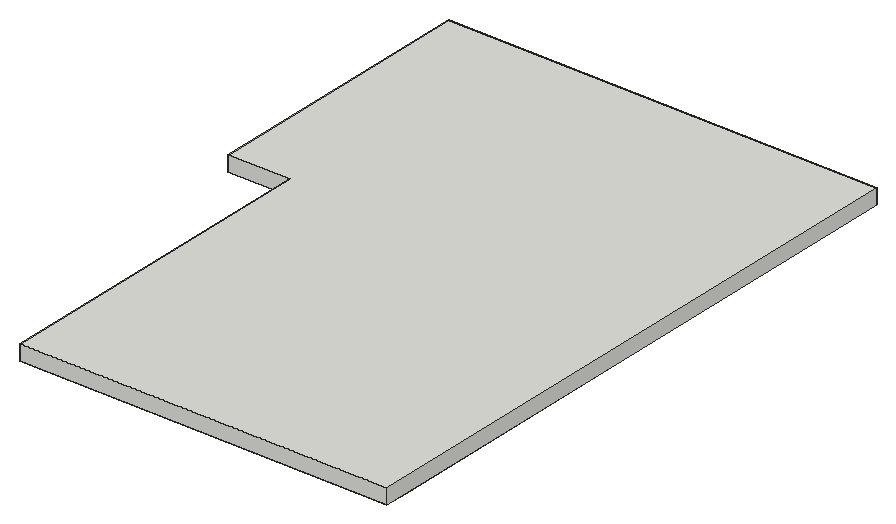
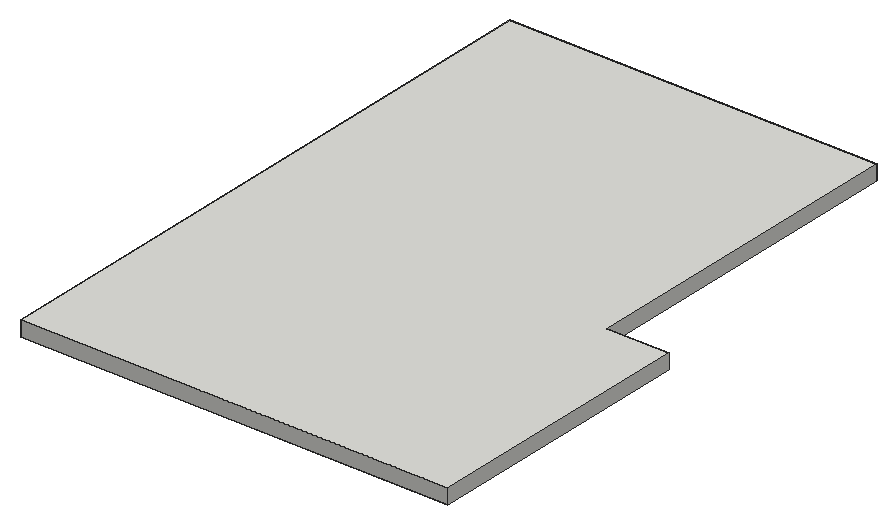
# SketchUp Ruby script. Lengths in inches.
U = 1.inch
M = Sketchup.active_model
def pt(a) = Geom::Point3d.new(a.map { |v| v * U })
def face(e, loops, mat)
  f = e.add_face(loops[0].map { |a| pt(a) })
  loops[1..].each { |l| e.add_face(l.map { |a| pt(a) }).erase! }
  f.material = f.back_material = mat if mat
  f
end
# faces: each face lists its corners as indices into pts; further lists are holes
def faces(e, pts, list, mat = nil) = list.each { |f| face(e, (f[0].is_a?(Array) ? f : [f]).map { |l| l.map { |i| pts[i] } }, mat) }
# xy, xz, yz: faces in a plane at the given z, y or x. An outline is a flat list of corners, or four numbers for a rectangle; further outlines are holes
def ring(l) = l.size == 4 ? [[l[0], l[1]], [l[2], l[1]], [l[2], l[3]], [l[0], l[3]]] : l.each_slice(2).to_a
def flat(e, list, mat, &to3) = list.each { |f| face(e, (f[0].is_a?(Array) ? f : [f]).map { |l| ring(l).map { |u, v| to3.(u, v) } }, mat) }
def xy(e, z, list, mat = nil) = flat(e, list, mat) { |x, y| [x, y, z] }
def xz(e, y, list, mat = nil) = flat(e, list, mat) { |x, z| [x, y, z] }
def yz(e, x, list, mat = nil) = flat(e, list, mat) { |y, z| [x, y, z] }
def lines(e, pts, list) = list.each { |a, b| e.add_line(pt(pts[a]), pt(pts[b])) }
# prism: a flat outline (further loops are holes) pulled along v
def prism(e, loops, v, mat = nil)
  f = face(e, loops, mat); d = Geom::Vector3d.new(v.map { |x| x * U })
  f.pushpull(f.normal.samedirection?(d) ? d.length : -d.length)
end
def box(e, o, s, mat = nil) = prism(e, [[o, [o[0] + s[0], o[1], o[2]], [o[0] + s[0], o[1] + s[1], o[2]], [o[0], o[1] + s[1], o[2]]]], [0, 0, s[2]], mat)
def at(x, y, z, deg = 0) = Geom::Transformation.translation(pt([x, y, z])) * Geom::Transformation.rotation(ORIGIN, Z_AXIS, deg.degrees)
def axes(o, x, y, z) = Geom::Transformation.new([*x, 0, *y, 0, *z, 0, *pt(o).to_a, 1])
def part(name) = M.definitions.add(name)
# library, detail: a bought-in or finely detailed component or shape, given as its bounding box
def library(name, o, s) = part(name).tap { |d| box(d.entities, o, s) }
def detail(e, o, s) = box(e.add_group.entities, o, s)
def put(e, d, t, mat = nil) = e.add_instance(d, t).tap { |i| i.material = mat if mat }
def group(e, t, mat = nil) = e.add_group.tap { |g| g.transformation = t; g.material = mat if mat }.entities
root = M.entities
M.materials.add("False ceiling Light").color = [250, 225, 158]
M.materials.add("[Wood Veneer 01]3").color = [120, 70, 37]
c1 = library("Group\#28",[0,0,0],[152,89,0.5])
c2 = library("Group\#27",[0,0,0],[125,62,0.75])
xy(root,121,[[[75.29,35.75,144.17,35.75,144.21,35.76,144.3,35.76,144.34,35.77,144.38,35.77,144.42,35.78,144.47,35.78,144.55,35.8,144.59,35.8,144.63,35.8125,144.68,35.82,144.92,35.88,144.96,35.9,145.04,35.92,145.08,35.9375,145.125,35.95,145.16,35.97,145.2,35.98,145.24,36,145.28,36.01,145.4,36.07,145.4375,36.09,145.48,36.1,145.51,36.125,145.55,36.14,145.59,36.16,145.625,36.1875,145.66,36.21,145.7,36.23,145.73,36.25,145.77,36.27,145.81,36.3,145.84,36.32,145.875,36.35,145.91,36.37,145.94,36.4,145.98,36.42,146.01,36.45,146.05,36.47,146.14,36.56,146.17,36.58,146.21,36.61,146.39,36.79,146.42,36.83,146.44,36.86,146.53,36.95,146.55,36.99,146.58,37.02,146.6,37.06,146.63,37.09,146.65,37.125,146.68,37.16,146.7,37.19,146.73,37.23,146.75,37.27,146.77,37.3,146.79,37.34,146.8125,37.375,146.84,37.41,146.86,37.45,146.875,37.49,146.9,37.52,146.91,37.5625,146.93,37.6,146.99,37.72,147,37.76,147.02,37.8,147.03,37.84,147.05,37.875,147.0625,37.92,147.08,37.96,147.1,38.04,147.12,38.08,147.18,38.32,147.1875,38.37,147.2,38.41,147.2,38.45,147.22,38.53,147.22,38.58,147.23,38.62,147.23,38.66,147.24,38.7,147.24,38.79,147.25,38.83,147.25,171.17,147.24,171.21,147.24,171.3,147.23,171.34,147.23,171.38,147.22,171.42,147.22,171.47,147.2,171.55,147.2,171.59,147.1875,171.63,147.18,171.68,147.12,171.92,147.1,171.96,147.08,172.04,147.0625,172.08,147.05,172.125,147.03,172.16,147.02,172.2,147,172.24,146.99,172.28,146.93,172.4,146.91,172.4375,146.9,172.48,146.875,172.51,146.86,172.55,146.84,172.59,146.8125,172.625,146.79,172.66,146.77,172.7,146.75,172.73,146.73,172.77,146.7,172.81,146.68,172.84,146.65,172.875,146.63,172.91,146.6,172.94,146.58,172.98,146.55,173.01,146.53,173.05,146.44,173.14,146.42,173.17,146.39,173.21,146.21,173.39,146.17,173.42,146.14,173.44,146.05,173.53,146.01,173.55,145.98,173.58,145.94,173.6,145.91,173.63,145.875,173.65,145.84,173.68,145.81,173.7,145.77,173.73,145.73,173.75,145.7,173.77,145.66,173.79,145.625,173.8125,145.59,173.84,145.55,173.86,145.51,173.875,145.48,173.9,145.4375,173.91,145.4,173.93,145.28,173.99,145.24,174,145.2,174.02,145.16,174.03,145.125,174.05,145.08,174.0625,145.04,174.08,144.96,174.1,144.92,174.12,144.68,174.18,144.63,174.1875,144.59,174.2,144.55,174.2,144.47,174.22,144.42,174.22,144.38,174.23,144.34,174.23,144.3,174.24,144.21,174.24,144.17,174.25,75.29,174.25,74.58,174.2,74.16,174.12,73.76,173.99,73.38,173.8,73.03,173.5625,72.72,173.28,72.4375,172.97,72.2,172.62,72.01,172.24,71.88,171.84,71.8,171.42,71.75,170.71,71.75,39.29,71.8,38.58,71.88,38.16,72.01,37.76,72.2,37.38,72.4375,37.03,72.72,36.72,73.03,36.4375,73.38,36.2,73.76,36.01,74.16,35.88,74.58,35.8],[92.62,42.5,91.86,42.54,91.67,42.5625,91.48,42.58,91.3,42.6,90.92,42.65,90.54,42.71,90.36,42.74,90.17,42.78,89.99,42.82,89.8,42.86,89.62,42.9,89.43,42.95,89.25,42.99,89.0625,43.04,88.88,43.1,88.7,43.15,88.16,43.33,87.98,43.4,87.8,43.46,87.45,43.6,87.28,43.68,87.1,43.75,86.76,43.91,86.59,44,86.42,44.08,85.91,44.35,85.75,44.44,85.59,44.54,85.42,44.64,84.94,44.94,84.79,45.05,84.63,45.16,84.48,45.27,84.32,45.38,84.17,45.5,84.02,45.61,83.73,45.85,83.58,45.97,83.4375,46.1,83.3,46.22,82.88,46.61,82.75,46.75,82.61,46.88,82.22,47.3,82.1,47.4375,81.97,47.58,81.85,47.73,81.61,48.02,81.5,48.17,81.38,48.32,81.27,48.48,81.16,48.63,81.05,48.79,80.94,48.94,80.64,49.42,80.54,49.59,80.44,49.75,80.35,49.91,80.08,50.42,80,50.59,79.91,50.76,79.75,51.1,79.68,51.28,79.6,51.45,79.46,51.8,79.4,51.98,79.33,52.16,79.15,52.7,79.1,52.88,79.04,53.0625,78.99,53.25,78.95,53.43,78.9,53.62,78.86,53.8,78.82,53.99,78.78,54.17,78.74,54.36,78.71,54.54,78.65,54.92,78.6,55.3,78.58,55.48,78.5625,55.67,78.54,55.86,78.5,56.62,78.5,153.38,78.54,154.14,78.5625,154.33,78.58,154.52,78.6,154.7,78.65,155.08,78.71,155.46,78.74,155.64,78.78,155.83,78.82,156.01,78.86,156.2,78.9,156.38,78.95,156.57,78.99,156.75,79.04,156.9375,79.1,157.12,79.15,157.3,79.33,157.84,79.4,158.02,79.46,158.2,79.6,158.55,79.68,158.72,79.75,158.9,79.91,159.24,80,159.41,80.08,159.58,80.35,160.09,80.44,160.25,80.54,160.41,80.64,160.58,80.94,161.06,81.05,161.21,81.16,161.37,81.27,161.52,81.38,161.68,81.5,161.83,81.61,161.98,81.85,162.27,81.97,162.42,82.1,162.5625,82.22,162.7,82.61,163.12,82.75,163.25,82.88,163.39,83.3,163.78,83.4375,163.9,83.58,164.03,83.73,164.15,84.02,164.39,84.17,164.5,84.32,164.62,84.48,164.73,84.63,164.84,84.79,164.95,84.94,165.06,85.42,165.36,85.59,165.46,85.75,165.56,85.91,165.65,86.42,165.92,86.59,166,86.76,166.09,87.1,166.25,87.28,166.32,87.45,166.4,87.8,166.54,87.98,166.6,88.16,166.67,88.7,166.85,88.88,166.9,89.0625,166.96,89.25,167.01,89.43,167.05,89.62,167.1,89.8,167.14,89.99,167.18,90.17,167.22,90.36,167.26,90.54,167.29,90.92,167.35,91.3,167.4,91.48,167.42,91.67,167.4375,91.86,167.46,92.62,167.5,126.38,167.5,127.14,167.46,127.33,167.4375,127.52,167.42,127.7,167.4,128.08,167.35,128.46,167.29,128.64,167.26,128.83,167.22,129.01,167.18,129.2,167.14,129.38,167.1,129.57,167.05,129.75,167.01,129.9375,166.96,130.12,166.9,130.3,166.85,130.84,166.67,131.02,166.6,131.2,166.54,131.55,166.4,131.72,166.32,131.9,166.25,132.24,166.09,132.41,166,132.58,165.92,133.09,165.65,133.25,165.56,133.41,165.46,133.58,165.36,134.06,165.06,134.21,164.95,134.37,164.84,134.52,164.73,134.68,164.62,134.83,164.5,134.98,164.39,135.27,164.15,135.42,164.03,135.5625,163.9,135.7,163.78,136.12,163.39,136.25,163.25,136.39,163.12,136.78,162.7,136.9,162.5625,137.03,162.42,137.15,162.27,137.39,161.98,137.5,161.83,137.62,161.68,137.73,161.52,137.84,161.37,137.95,161.21,138.06,161.06,138.36,160.58,138.46,160.41,138.56,160.25,138.65,160.09,138.92,159.58,139,159.41,139.09,159.24,139.25,158.9,139.32,158.72,139.4,158.55,139.54,158.2,139.6,158.02,139.67,157.84,139.85,157.3,139.9,157.12,139.96,156.9375,140.01,156.75,140.05,156.57,140.1,156.38,140.14,156.2,140.18,156.01,140.22,155.83,140.26,155.64,140.29,155.46,140.35,155.08,140.4,154.7,140.42,154.52,140.4375,154.33,140.46,154.14,140.5,153.38,140.5,56.62,140.46,55.86,140.4375,55.67,140.42,55.48,140.4,55.3,140.35,54.92,140.29,54.54,140.26,54.36,140.22,54.17,140.18,53.99,140.14,53.8,140.1,53.62,140.05,53.43,140.01,53.25,139.96,53.0625,139.9,52.88,139.85,52.7,139.67,52.16,139.6,51.98,139.54,51.8,139.4,51.45,139.32,51.28,139.25,51.1,139.09,50.76,139,50.59,138.92,50.42,138.65,49.91,138.56,49.75,138.46,49.59,138.36,49.42,138.06,48.94,137.95,48.79,137.84,48.63,137.73,48.48,137.62,48.32,137.5,48.17,137.39,48.02,137.15,47.73,137.03,47.58,136.9,47.4375,136.78,47.3,136.39,46.88,136.25,46.75,136.12,46.61,135.7,46.22,135.5625,46.1,135.42,45.97,135.27,45.85,134.98,45.61,134.83,45.5,134.68,45.38,134.52,45.27,134.37,45.16,134.21,45.05,134.06,44.94,133.58,44.64,133.41,44.54,133.25,44.44,133.09,44.35,132.58,44.08,132.41,44,132.24,43.91,131.9,43.75,131.72,43.68,131.55,43.6,131.2,43.46,131.02,43.4,130.84,43.33,130.3,43.15,130.12,43.1,129.9375,43.04,129.75,42.99,129.57,42.95,129.38,42.9,129.2,42.86,129.01,42.82,128.83,42.78,128.64,42.74,128.46,42.71,128.08,42.65,127.7,42.6,127.52,42.58,127.33,42.5625,127.14,42.54,126.38,42.5]]])
xy(root,126,[[24,0,24,132,0,132,0,240,168,240,168,231,9,231,9,141,33,141,33,9,168,9,168,0],[33,9,33,141,9,141,9,231,168,231,168,9]])
xy(root,132,[[24,0,168,0,168,240,0,240,0,132,24,132]])
xz(root,0,[[24,126,168,132]])
xz(root,132,[[0,126,24,132]])
xz(root,166.5,[[92.65,121,92.82,121.5],[92.82,121,93,121.5],[93,121,126,121.5],[126,121,126.18,121.5],[126.18,121,126.35,121.5]],"[Wood Veneer 01]3")
xz(root,174.25,[[75.29,121,143.97,123]])
xz(root,176.25,[[75.22,121,143.98,123]])
xz(root,240,[[0,126,168,132]])
yz(root,0,[[132,126,240,132]])
yz(root,24,[[0,126,132,132]])
yz(root,79.5,[[153,121,153.18,121.5],[153.18,121,153.35,121.5]],"[Wood Veneer 01]3")
yz(root,168,[[0,126,240,132]])
p = [[79.51,153.53,121],[79.5,153.35,121],[79.5,153.35,121.5],[79.51,153.53,121.5],[79.52,153.71,121],[79.52,153.71,121.5],
  [79.53,153.88,121],[79.53,153.88,121.5],[79.54,154.06,121],[79.54,154.06,121.5],[79.56,154.24,121],[79.56,154.24,121.5],
  [79.57,154.41,121],[79.57,154.41,121.5],[79.59,154.59,121],[79.59,154.59,121.5],[79.62,154.76,121],[79.62,154.76,121.5],
  [79.64,154.9375,121],[79.64,154.9375,121.5],[79.67,155.11,121],[79.67,155.11,121.5],[79.69,155.29,121],[79.69,155.29,121.5],
  [79.73,155.46,121],[79.73,155.46,121.5],[79.76,155.63,121],[79.76,155.63,121.5],[79.79,155.81,121],[79.79,155.81,121.5],
  [139.24,155.63,121],[139.21,155.81,121],[139.21,155.81,121.5],[139.24,155.63,121.5],[79.83,155.98,121],[79.83,155.98,121.5],
  [139.17,155.98,121],[139.17,155.98,121.5],[79.87,156.15,121],[79.87,156.15,121.5],[139.13,156.15,121],[139.13,156.15,121.5],
  [79.92,156.32,121],[79.92,156.32,121.5],[139.08,156.32,121],[139.08,156.32,121.5],[79.96,156.49,121],[79.96,156.49,121.5],
  [139.04,156.49,121],[139.04,156.49,121.5],[80.01,156.66,121],[80.01,156.66,121.5],[138.99,156.66,121],[138.99,156.66,121.5],
  [80.06,156.83,121],[80.06,156.83,121.5],[138.94,156.83,121],[138.94,156.83,121.5],[80.11,157,121],[80.11,157,121.5],
  [138.89,157,121],[138.89,157,121.5],[80.16,157.17,121],[80.16,157.17,121.5],[138.84,157.17,121],[138.84,157.17,121.5],
  [80.22,157.34,121],[80.22,157.34,121.5],[138.78,157.34,121],[138.78,157.34,121.5],[80.27,157.51,121],[80.27,157.51,121.5],
  [138.73,157.51,121],[138.73,157.51,121.5],[80.33,157.67,121],[80.33,157.67,121.5],[138.67,157.67,121],[138.67,157.67,121.5],
  [80.4,157.84,121],[80.4,157.84,121.5],[138.6,157.84,121],[138.6,157.84,121.5],[80.46,158,121],[80.46,158,121.5],
  [138.54,158,121],[138.54,158,121.5],[80.53,158.17,121],[80.53,158.17,121.5],[138.47,158.17,121],[138.47,158.17,121.5],
  [80.6,158.33,121],[80.6,158.33,121.5],[138.4,158.33,121],[138.4,158.33,121.5],[80.67,158.49,121],[80.67,158.49,121.5],
  [138.33,158.49,121],[138.33,158.49,121.5],[80.74,158.65,121],[80.74,158.65,121.5],[138.26,158.65,121],[138.26,158.65,121.5],
  [80.82,158.8125,121],[80.82,158.8125,121.5],[138.18,158.8125,121],[138.18,158.8125,121.5],[80.89,158.97,121],[80.89,158.97,121.5],
  [138.11,158.97,121],[138.11,158.97,121.5],[80.97,159.13,121],[80.97,159.13,121.5],[138.03,159.13,121],[138.03,159.13,121.5],
  [81.05,159.29,121],[81.05,159.29,121.5],[137.95,159.29,121],[137.95,159.29,121.5],[81.14,159.44,121],[81.14,159.44,121.5],
  [137.86,159.44,121],[137.86,159.44,121.5],[81.22,159.6,121],[81.22,159.6,121.5],[137.78,159.6,121],[137.78,159.6,121.5],
  [81.31,159.75,121],[81.31,159.75,121.5],[137.69,159.75,121],[137.69,159.75,121.5],[81.4,159.9,121],[81.4,159.9,121.5],
  [137.6,159.9,121],[137.6,159.9,121.5],[81.49,160.05,121],[81.49,160.05,121.5],[137.51,160.05,121],[137.51,160.05,121.5],
  [81.58,160.2,121],[81.58,160.2,121.5],[137.42,160.2,121],[137.42,160.2,121.5],[81.68,160.35,121],[81.68,160.35,121.5],
  [137.32,160.35,121],[137.32,160.35,121.5],[81.78,160.5,121],[81.78,160.5,121.5],[137.22,160.5,121],[137.22,160.5,121.5],
  [81.875,160.65,121],[81.875,160.65,121.5],[137.125,160.65,121],[137.125,160.65,121.5],[81.98,160.79,121],[81.98,160.79,121.5],
  [137.02,160.79,121],[137.02,160.79,121.5],[82.08,160.94,121],[82.08,160.94,121.5],[136.92,160.94,121],[136.92,160.94,121.5],
  [82.18,161.08,121],[82.18,161.08,121.5],[136.82,161.08,121],[136.82,161.08,121.5],[82.29,161.22,121],[82.29,161.22,121.5],
  [136.71,161.22,121],[136.71,161.22,121.5],[82.4,161.36,121],[82.4,161.36,121.5],[136.6,161.36,121],[136.6,161.36,121.5],
  [82.51,161.5,121],[82.51,161.5,121.5],[136.49,161.5,121],[136.49,161.5,121.5],[82.62,161.63,121],[82.62,161.63,121.5],
  [136.38,161.63,121],[136.38,161.63,121.5],[82.73,161.77,121],[82.73,161.77,121.5],[136.27,161.77,121],[136.27,161.77,121.5],
  [82.85,161.9,121],[82.85,161.9,121.5],[136.15,161.9,121],[136.15,161.9,121.5],[82.97,162.03,121],[82.97,162.03,121.5],
  [136.03,162.03,121],[136.03,162.03,121.5],[83.09,162.16,121],[83.09,162.16,121.5],[135.91,162.16,121],[135.91,162.16,121.5],
  [83.21,162.29,121],[83.21,162.29,121.5],[135.79,162.29,121],[135.79,162.29,121.5],[83.33,162.42,121],[83.33,162.42,121.5],
  [135.67,162.42,121],[135.67,162.42,121.5],[83.45,162.55,121],[83.45,162.55,121.5],[135.55,162.55,121],[135.55,162.55,121.5],
  [83.58,162.67,121],[83.58,162.67,121.5],[135.42,162.67,121],[135.42,162.67,121.5],[83.71,162.79,121],[83.71,162.79,121.5],
  [135.29,162.79,121],[135.29,162.79,121.5],[83.84,162.91,121],[83.84,162.91,121.5],[135.16,162.91,121],[135.16,162.91,121.5],
  [83.97,163.03,121],[83.97,163.03,121.5],[135.03,163.03,121],[135.03,163.03,121.5],[84.1,163.15,121],[84.1,163.15,121.5],
  [134.9,163.15,121],[134.9,163.15,121.5],[84.23,163.27,121],[84.23,163.27,121.5],[134.77,163.27,121],[134.77,163.27,121.5],
  [84.37,163.38,121],[84.37,163.38,121.5],[134.63,163.38,121],[134.63,163.38,121.5],[84.5,163.49,121],[84.5,163.49,121.5],
  [134.5,163.49,121],[134.5,163.49,121.5],[84.64,163.6,121],[84.64,163.6,121.5],[134.36,163.6,121],[134.36,163.6,121.5],
  [84.78,163.71,121],[84.78,163.71,121.5],[134.22,163.71,121],[134.22,163.71,121.5],[84.92,163.82,121],[84.92,163.82,121.5],
  [134.08,163.82,121],[134.08,163.82,121.5],[85.06,163.92,121],[85.06,163.92,121.5],[133.94,163.92,121],[133.94,163.92,121.5],
  [85.21,164.02,121],[85.21,164.02,121.5],[133.79,164.02,121],[133.79,164.02,121.5],[85.35,164.125,121],[85.35,164.125,121.5],
  [133.65,164.125,121],[133.65,164.125,121.5],[85.5,164.22,121],[85.5,164.22,121.5],[133.5,164.22,121],[133.5,164.22,121.5],
  [85.65,164.32,121],[85.65,164.32,121.5],[133.35,164.32,121],[133.35,164.32,121.5],[85.8,164.42,121],[85.8,164.42,121.5],
  [133.2,164.42,121],[133.2,164.42,121.5],[85.95,164.51,121],[85.95,164.51,121.5],[133.05,164.51,121],[133.05,164.51,121.5],
  [86.1,164.6,121],[86.1,164.6,121.5],[132.9,164.6,121],[132.9,164.6,121.5],[86.25,164.69,121],[86.25,164.69,121.5],
  [132.75,164.69,121],[132.75,164.69,121.5],[86.4,164.78,121],[86.4,164.78,121.5],[132.6,164.78,121],[132.6,164.78,121.5],
  [86.56,164.86,121],[86.56,164.86,121.5],[132.44,164.86,121],[132.44,164.86,121.5],[86.71,164.95,121],[86.71,164.95,121.5],
  [86.87,165.03,121],[86.87,165.03,121.5],[132.29,164.95,121],[132.13,165.03,121],[132.13,165.03,121.5],[132.29,164.95,121.5],
  [87.03,165.11,121],[87.03,165.11,121.5],[131.97,165.11,121],[131.97,165.11,121.5],[87.1875,165.18,121],[87.1875,165.18,121.5],
  [131.8125,165.18,121],[131.8125,165.18,121.5],[87.35,165.26,121],[87.35,165.26,121.5],[131.65,165.26,121],[131.65,165.26,121.5],
  [87.51,165.33,121],[87.51,165.33,121.5],[87.67,165.4,121],[87.67,165.4,121.5],[131.49,165.33,121],[131.33,165.4,121],
  [131.33,165.4,121.5],[131.49,165.33,121.5],[87.83,165.47,121],[87.83,165.47,121.5],[131.17,165.47,121],[131.17,165.47,121.5],
  [88,165.54,121],[88,165.54,121.5],[88.16,165.6,121],[88.16,165.6,121.5],[131,165.54,121],[130.84,165.6,121],
  [130.84,165.6,121.5],[131,165.54,121.5],[88.33,165.67,121],[88.33,165.67,121.5],[130.67,165.67,121],[130.67,165.67,121.5],
  [88.49,165.73,121],[88.49,165.73,121.5],[88.66,165.78,121],[88.66,165.78,121.5],[130.51,165.73,121],[130.34,165.78,121],
  [130.34,165.78,121.5],[130.51,165.73,121.5],[88.83,165.84,121],[88.83,165.84,121.5],[89,165.89,121],[89,165.89,121.5],
  [130.17,165.84,121],[130,165.89,121],[130,165.89,121.5],[130.17,165.84,121.5],[89.17,165.94,121],[89.17,165.94,121.5],
  [89.34,165.99,121],[89.34,165.99,121.5],[129.83,165.94,121],[129.66,165.99,121],[129.66,165.99,121.5],[129.83,165.94,121.5],
  [89.51,166.04,121],[89.51,166.04,121.5],[89.68,166.08,121],[89.68,166.08,121.5],[129.49,166.04,121],[129.32,166.08,121],
  [129.32,166.08,121.5],[129.49,166.04,121.5],[89.85,166.13,121],[89.85,166.13,121.5],[90.02,166.17,121],[90.02,166.17,121.5],
  [129.15,166.13,121],[128.98,166.17,121],[128.98,166.17,121.5],[129.15,166.13,121.5],[90.19,166.21,121],[90.19,166.21,121.5],
  [90.37,166.24,121],[90.37,166.24,121.5],[90.54,166.27,121],[90.54,166.27,121.5],[128.63,166.24,121],[128.46,166.27,121],
  [128.46,166.27,121.5],[128.63,166.24,121.5],[128.81,166.21,121],[128.81,166.21,121.5],[90.71,166.31,121],[90.71,166.31,121.5],
  [90.89,166.33,121],[90.89,166.33,121.5],[91.0625,166.36,121],[91.0625,166.36,121.5],[128.11,166.33,121],[127.9375,166.36,121],
  [127.9375,166.36,121.5],[128.11,166.33,121.5],[128.29,166.31,121],[128.29,166.31,121.5],[91.24,166.38,121],[91.24,166.38,121.5],
  [91.41,166.41,121],[91.41,166.41,121.5],[91.59,166.43,121],[91.59,166.43,121.5],[91.76,166.44,121],[91.76,166.44,121.5],
  [91.94,166.46,121],[91.94,166.46,121.5],[127.24,166.44,121],[127.06,166.46,121],[127.06,166.46,121.5],[127.24,166.44,121.5],
  [127.41,166.43,121],[127.41,166.43,121.5],[127.59,166.41,121],[127.59,166.41,121.5],[127.76,166.38,121],[127.76,166.38,121.5],
  [92.12,166.47,121],[92.12,166.47,121.5],[92.29,166.48,121],[92.29,166.48,121.5],[92.47,166.49,121],[92.47,166.49,121.5],
  [92.65,166.5,121],[92.65,166.5,121.5],[126.53,166.49,121],[126.35,166.5,121],[126.35,166.5,121.5],[126.53,166.49,121.5],
  [126.71,166.48,121],[126.71,166.48,121.5],[126.88,166.47,121],[126.88,166.47,121.5],[71.75,170.71,121],[71.8,171.42,121],
  [71.8,171.42,123],[71.75,170.71,123],[69.81,171.68,121],[69.75,170.78,121],[69.75,170.78,123],[69.81,171.68,123],
  [71.88,171.84,121],[71.88,171.84,123],[69.94,172.36,121],[69.94,172.36,123],[72.01,172.24,121],[72.01,172.24,123],
  [72.2,172.62,121],[72.2,172.62,123],[70.16,173,121],[70.16,173,123],[72.4375,172.97,121],[72.4375,172.97,123],
  [70.47,173.62,121],[70.47,173.62,123],[72.72,173.28,121],[72.72,173.28,123],[73.03,173.5625,121],[73.03,173.5625,123],
  [70.85,174.1875,121],[70.85,174.1875,123],[73.38,173.8,121],[73.38,173.8,123],[73.76,173.99,121],[73.76,173.99,123],
  [74.16,174.12,121],[74.16,174.12,123],[74.58,174.2,121],[74.58,174.2,123],[71.3,174.7,121],[71.3,174.7,123],
  [75.29,174.25,121],[75.29,174.25,123],[71.8125,175.15,121],[71.8125,175.15,123],[72.38,175.53,121],[72.38,175.53,123],
  [73,175.84,121],[73,175.84,123],[73.64,176.06,121],[73.64,176.06,123],[74.32,176.19,121],[74.32,176.19,123],
  [75.22,176.25,121],[75.22,176.25,123]]
faces(root,p,[[0,1,2,3],[4,0,3,5],[6,4,5,7],[8,6,7,9],[10,8,9,11],[12,10,11,13],[14,12,13,15],[16,14,15,17],
  [18,16,17,19],[20,18,19,21],[22,20,21,23],[24,22,23,25],[26,24,25,27],[28,26,27,29],[30,31,32,33],[34,28,29,35],
  [31,36,37,32],[38,34,35,39],[36,40,41,37],[42,38,39,43],[40,44,45,41],[46,42,43,47],[44,48,49,45],[50,46,47,51],
  [48,52,53,49],[54,50,51,55],[52,56,57,53],[58,54,55,59],[56,60,61,57],[62,58,59,63],[60,64,65,61],[66,62,63,67],
  [64,68,69,65],[70,66,67,71],[68,72,73,69],[74,70,71,75],[72,76,77,73],[78,74,75,79],[76,80,81,77],[82,78,79,83],
  [80,84,85,81],[86,82,83,87],[84,88,89,85],[90,86,87,91],[88,92,93,89],[94,90,91,95],[92,96,97,93],[98,94,95,99],
  [96,100,101,97],[102,98,99,103],[100,104,105,101],[106,102,103,107],[104,108,109,105],[110,106,107,111],[108,112,113,109],[114,110,111,115],
  [112,116,117,113],[118,114,115,119],[116,120,121,117],[122,118,119,123],[120,124,125,121],[126,122,123,127],[124,128,129,125],[130,126,127,131],
  [128,132,133,129],[134,130,131,135],[132,136,137,133],[138,134,135,139],[136,140,141,137],[142,138,139,143],[140,144,145,141],[146,142,143,147],
  [144,148,149,145],[150,146,147,151],[148,152,153,149],[154,150,151,155],[152,156,157,153],[158,154,155,159],[156,160,161,157],[162,158,159,163],
  [160,164,165,161],[166,162,163,167],[164,168,169,165],[170,166,167,171],[168,172,173,169],[174,170,171,175],[172,176,177,173],[178,174,175,179],
  [176,180,181,177],[182,178,179,183],[180,184,185,181],[186,182,183,187],[184,188,189,185],[190,186,187,191],[188,192,193,189],[194,190,191,195],
  [192,196,197,193],[198,194,195,199],[196,200,201,197],[202,198,199,203],[200,204,205,201],[206,202,203,207],[204,208,209,205],[210,206,207,211],
  [208,212,213,209],[214,210,211,215],[212,216,217,213],[218,214,215,219],[216,220,221,217],[222,218,219,223],[220,224,225,221],[226,222,223,227],
  [224,228,229,225],[230,226,227,231],[228,232,233,229],[234,230,231,235],[232,236,237,233],[238,234,235,239],[236,240,241,237],[242,238,239,243],
  [240,244,245,241],[246,242,243,247],[244,248,249,245],[250,246,247,251],[248,252,253,249],[254,250,251,255],[252,256,257,253],[258,254,255,259],
  [256,260,261,257],[262,258,259,263],[260,264,265,261],[266,262,263,267],[264,268,269,265],[270,266,267,271],[268,272,273,269],[274,270,271,275],
  [272,276,277,273],[278,274,275,279],[276,280,281,277],[282,278,279,283],[280,284,285,281],[286,282,283,287],[284,288,289,285],[290,286,287,291],
  [288,292,293,289],[294,290,291,295],[292,296,297,293],[298,294,295,299],[300,298,299,301],[302,303,304,305],[296,302,305,297],[306,300,301,307],
  [303,308,309,304],[310,306,307,311],[308,312,313,309],[314,310,311,315],[312,316,317,313],[318,314,315,319],[320,318,319,321],[322,323,324,325],
  [316,322,325,317],[326,320,321,327],[323,328,329,324],[330,326,327,331],[332,330,331,333],[334,335,336,337],[328,334,337,329],[338,332,333,339],
  [335,340,341,336],[342,338,339,343],[344,342,343,345],[346,347,348,349],[340,346,349,341],[350,344,345,351],[352,350,351,353],[354,355,356,357],
  [347,354,357,348],[358,352,353,359],[360,358,359,361],[362,363,364,365],[355,362,365,356],[366,360,361,367],[368,366,367,369],[370,371,372,373],
  [363,370,373,364],[374,368,369,375],[376,374,375,377],[378,379,380,381],[371,378,381,372],[382,376,377,383],[384,382,383,385],[386,384,385,387],
  [388,389,390,391],[392,388,391,393],[379,392,393,380],[394,386,387,395],[396,394,395,397],[398,396,397,399],[400,401,402,403],[404,400,403,405],
  [389,404,405,390],[406,398,399,407],[408,406,407,409],[410,408,409,411],[412,410,411,413],[414,412,413,415],[416,417,418,419],[420,416,419,421],
  [422,420,421,423],[424,422,423,425],[401,424,425,402],[426,414,415,427],[428,426,427,429],[430,428,429,431],[432,430,431,433],[434,435,436,437],
  [438,434,437,439],[440,438,439,441],[417,440,441,418]],"[Wood Veneer 01]3")
faces(root,p,[[442,443,444,445],[446,447,448,449],[443,450,451,444],[452,446,449,453],[450,454,455,451],[454,456,457,455],[458,452,453,459],[456,460,461,457],
  [462,458,459,463],[460,464,465,461],[464,466,467,465],[468,462,463,469],[466,470,471,467],[470,472,473,471],[472,474,475,473],[474,476,477,475],
  [478,468,469,479],[476,480,481,477],[482,478,479,483],[484,482,483,485],[486,484,485,487],[488,486,487,489],[490,488,489,491],[492,490,491,493]])
g1 = group(root,at(162,21,123.25,90),"False ceiling Light")
prism(g1,[[[0,3,-0.25],[0,122.75,-0.25],[126.5,122.75,-0.25],[126.5,141,-0.25],[179.97,141,-0.25],[179.97,0,-0.25],[0,0,-0.25]],[[0.5,122.25,-0.25],[0.5,3,-0.25],[0.5,0.5,-0.25],[179.47,0.5,-0.25],[179.47,140.5,-0.25],[127,140.5,-0.25],[127,122.25,-0.25]]],[0,0,0.25])
put(root,c1,at(154,29,121,90),"False ceiling Light")
put(root,c2,at(140.5,42.5,121,90),"False ceiling Light")
